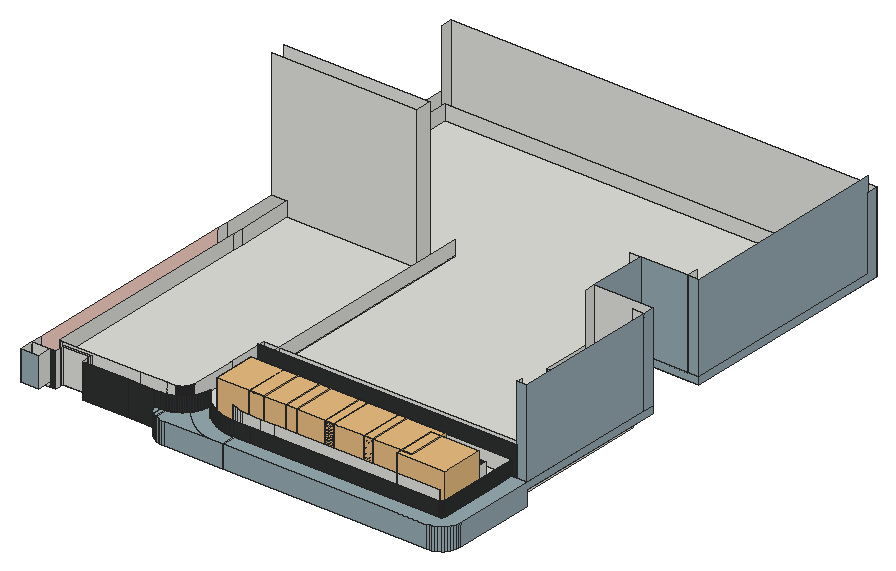
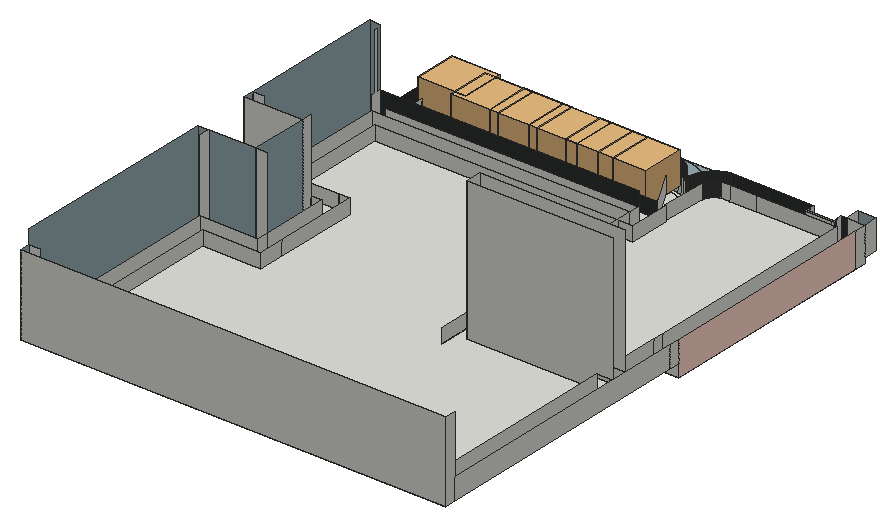
# SketchUp Ruby script. Lengths in inches.
U = 1.inch
M = Sketchup.active_model
def pt(a) = Geom::Point3d.new(a.map { |v| v * U })
def face(e, loops, mat)
  f = e.add_face(loops[0].map { |a| pt(a) })
  loops[1..].each { |l| e.add_face(l.map { |a| pt(a) }).erase! }
  f.material = f.back_material = mat if mat
  f
end
# faces: each face lists its corners as indices into pts; further lists are holes
def faces(e, pts, list, mat = nil) = list.each { |f| face(e, (f[0].is_a?(Array) ? f : [f]).map { |l| l.map { |i| pts[i] } }, mat) }
# xy, xz, yz: faces in a plane at the given z, y or x. An outline is a flat list of corners, or four numbers for a rectangle; further outlines are holes
def ring(l) = l.size == 4 ? [[l[0], l[1]], [l[2], l[1]], [l[2], l[3]], [l[0], l[3]]] : l.each_slice(2).to_a
def flat(e, list, mat, &to3) = list.each { |f| face(e, (f[0].is_a?(Array) ? f : [f]).map { |l| ring(l).map { |u, v| to3.(u, v) } }, mat) }
def xy(e, z, list, mat = nil) = flat(e, list, mat) { |x, y| [x, y, z] }
def xz(e, y, list, mat = nil) = flat(e, list, mat) { |x, z| [x, y, z] }
def yz(e, x, list, mat = nil) = flat(e, list, mat) { |y, z| [x, y, z] }
def lines(e, pts, list) = list.each { |a, b| e.add_line(pt(pts[a]), pt(pts[b])) }
# prism: a flat outline (further loops are holes) pulled along v
def prism(e, loops, v, mat = nil)
  f = face(e, loops, mat); d = Geom::Vector3d.new(v.map { |x| x * U })
  f.pushpull(f.normal.samedirection?(d) ? d.length : -d.length)
end
def box(e, o, s, mat = nil) = prism(e, [[o, [o[0] + s[0], o[1], o[2]], [o[0] + s[0], o[1] + s[1], o[2]], [o[0], o[1] + s[1], o[2]]]], [0, 0, s[2]], mat)
def at(x, y, z, deg = 0) = Geom::Transformation.translation(pt([x, y, z])) * Geom::Transformation.rotation(ORIGIN, Z_AXIS, deg.degrees)
def axes(o, x, y, z) = Geom::Transformation.new([*x, 0, *y, 0, *z, 0, *pt(o).to_a, 1])
def part(name) = M.definitions.add(name)
# library, detail: a bought-in or finely detailed component or shape, given as its bounding box
def library(name, o, s) = part(name).tap { |d| box(d.entities, o, s) }
def detail(e, o, s) = box(e.add_group.entities, o, s)
def put(e, d, t, mat = nil) = e.add_instance(d, t).tap { |i| i.material = mat if mat }
def group(e, t, mat = nil) = e.add_group.tap { |g| g.transformation = t; g.material = mat if mat }.entities
root = M.entities
M.materials.add("Generic").color = [150, 171, 178]
M.materials.add("Generic\#1").color = [47, 50, 50]
M.materials.add("[Color B01]").color = [255, 216, 204]
c1 = library("Tlon Light 650 Ceiling 152 007",[-12.8,-12.8,-3.78],[25.6,25.6,3.58])
c2 = library("Erigeron glaucus 004",[-15.59,-14.45,0.01],[31.39,28.46,21.32])
xy(root,360,[[129.04,30.0625,127.13,30.16,125.24,30.4375,123.38,30.9,121.58,31.54,120.21,32.1875,120.21,35.14,121.14,34.74,122.16,34.4,123.21,34.14,124.25,33.77,125.82,33.38,127.42,33.15,129.11,33.0625,176.86,33.0625,176.86,30.0625],[176.86,30.0625,176.86,33.0625,345.32,33.0625,347.08,33.18,348.73,33.5,349.22,33.67,349.85,33.71,350.48,33.8125,351.09,33.97,351.69,34.19,352.22,34.44,352.22,31.64,351.46,31.27,349.5,30.6,347.48,30.2,345.41,30.0625],[352.22,31.64,352.22,34.44,352.26,34.46,352.81,34.79,353.32,35.17,353.79,35.59,354.22,36.0625,354.6,36.57,354.9375,37.11,355.22,37.68,355.57,38.08,356.5,39.47,357.24,40.97,357.78,42.55,358.1,44.2,358.22,45.96,358.22,114.0625,361.22,114.0625,361.22,45.87,361.08,43.8,360.68,41.78,360.01,39.82,359.1,37.96,357.95,36.25,356.59,34.69,355.03,33.33,353.32,32.18],[120.21,32.1875,119.85,32.36,118.21,33.34,116.67,34.47,116.2,34.9,116.2,38.05,116.61,37.62,117.42,36.9,118.28,36.25,119.19,35.67,120.15,35.16,120.21,35.14],[116.2,34.9,115.25,35.75,113.97,37.17,112.82,38.7,111.84,40.34,111.01,42.0625,113.61,42.0625,114.06,41.08,114.59,40.14,115.19,39.25,115.87,38.4,116.2,38.05]])
xy(root,362,[[179.86,33.0625,179.86,44.93,173.27,45.23,169.71,45.72,166.21,46.54,162.8,47.67,159.51,49.1,156.36,50.83,153.39,52.85,150.61,55.12,148.05,57.64,145.73,60.38,143.67,63.33,136.45,75.96,136.2,64.13,136.13,63.2,136.03,62.26,135.875,61.33,135.68,60.41,135.45,59.5,135.17,58.6,134.85,57.72,134.5,56.85,134.1,56,133.66,55.16,133.1875,54.35,132.68,53.5625,132.13,52.8,131.55,52.06,130.93,51.35,130.28,50.67,129.61,50.01,128.9,49.39,128.16,48.81,127.4,48.26,126.61,47.74,125.81,47.26,124.98,46.82,124.125,46.42,123.26,46.05,122.375,45.73,121.48,45.45,120.57,45.21,119.2,44.91,119.2,45.0625,51.93,45.0625,51.93,51.0625,29.81,51.0625,29.81,45.0625,13.22,45.0625,13.22,231.0625,139.22,231.0625,139.22,126.0625,136.22,126.0625,136.22,111.0625,349.22,111.0625,349.22,33.67,348.73,33.5,347.08,33.18,345.32,33.0625],[176.86,33.0625,176.86,42.0625,173,42.24,169.17,42.77,165.4,43.64,161.73,44.86,158.1875,46.41,154.8,48.27,151.6,50.4375,148.6,52.89,145.85,55.6,143.35,58.55,141.14,61.72,139.22,65.08,139.19,64,139.12,62.92,139,61.85,138.83,60.79,138.61,59.73,138.34,58.6875,138.02,57.66,137.65,56.64,137.24,55.64,136.79,54.67,136.29,53.71,135.74,52.78,135.16,51.87,134.53,51,133.86,50.15,133.15,49.33,132.41,48.55,131.63,47.8,130.82,47.09,129.98,46.42,129.11,45.79,128.2,45.19,127.28,44.64,126.32,44.14,125.35,43.68,124.35,43.26,123.34,42.89,122.3125,42.57,121.27,42.29,120.21,42.0625,120.21,35.14,120.15,35.16,119.19,35.67,118.28,36.25,117.42,36.9,116.61,37.62,116.2,38.05,116.2,42.0625,51.93,42.0625,51.93,45.0625,119.2,45.0625,119.2,44.91,120.57,45.21,121.48,45.45,122.375,45.73,123.26,46.05,124.125,46.42,124.98,46.82,125.81,47.26,126.61,47.74,127.4,48.26,128.16,48.81,128.9,49.39,129.61,50.01,130.28,50.67,130.93,51.35,131.55,52.06,132.13,52.8,132.68,53.5625,133.1875,54.35,133.66,55.16,134.1,56,134.5,56.85,134.85,57.72,135.17,58.6,135.45,59.5,135.68,60.41,135.875,61.33,136.03,62.26,136.13,63.2,136.2,64.13,136.45,75.96,143.67,63.33,145.73,60.38,148.05,57.64,150.61,55.12,153.39,52.85,156.36,50.83,159.51,49.1,162.8,47.67,166.21,46.54,169.71,45.72,173.27,45.23,179.86,44.93,179.86,33.0625],[173.86,33.0625,173.86,39.2,172.72,39.25,168.62,39.82,164.59,40.75,160.66,42.06,156.86,43.71,153.23,45.71,149.8,48.03,146.6,50.65,143.65,53.56,140.97,56.72,140.9,56.82,140.45,55.5625,139.99,54.4375,139.48,53.33,138.91,52.26,138.3,51.2,137.64,50.18,136.93,49.19,136.17,48.24,135.38,47.32,134.54,46.43,133.66,45.59,132.75,44.79,131.8,44.03,130.81,43.32,129.79,42.65,128.75,42.03,127.67,41.46,126.57,40.94,125.45,40.47,124.31,40.05,123.21,39.7,123.21,34.14,122.16,34.4,121.14,34.74,120.21,35.14,120.21,42.0625,121.27,42.29,122.3125,42.57,123.34,42.89,124.35,43.26,125.35,43.68,126.32,44.14,127.28,44.64,128.2,45.19,129.11,45.79,129.98,46.42,130.82,47.09,131.63,47.8,132.41,48.55,133.15,49.33,133.86,50.15,134.53,51,135.16,51.87,135.74,52.78,136.29,53.71,136.79,54.67,137.24,55.64,137.65,56.64,138.02,57.66,138.34,58.6875,138.61,59.73,138.83,60.79,139,61.85,139.12,62.92,139.19,64,139.22,65.08,141.14,61.72,143.35,58.55,145.85,55.6,148.6,52.89,151.6,50.4375,154.8,48.27,158.1875,46.41,161.73,44.86,165.4,43.64,169.17,42.77,173,42.24,176.86,42.0625,176.86,33.0625],[129.11,33.0625,127.42,33.15,125.82,33.38,124.25,33.77,123.21,34.14,123.21,39.7,124.31,40.05,125.45,40.47,126.57,40.94,127.67,41.46,128.75,42.03,129.79,42.65,130.81,43.32,131.8,44.03,132.75,44.79,133.66,45.59,134.54,46.43,135.38,47.32,136.17,48.24,136.93,49.19,137.64,50.18,138.3,51.2,138.91,52.26,139.48,53.33,139.99,54.4375,140.45,55.5625,140.9,56.82,140.97,56.72,143.65,53.56,146.6,50.65,149.8,48.03,153.23,45.71,156.86,43.71,160.66,42.06,164.59,40.75,168.62,39.82,172.72,39.25,173.86,39.2,173.86,33.0625],[349.22,33.67,349.22,111.0625,136.22,111.0625,136.22,126.0625,139.22,126.0625,139.22,114.0625,352.22,114.0625,352.22,34.44,351.69,34.19,351.09,33.97,350.48,33.8125,349.85,33.71],
  [352.22,34.44,352.22,114.0625,358.22,114.0625,358.22,111.0625,355.22,111.0625,355.22,37.68,354.9375,37.11,354.6,36.57,354.22,36.0625,353.79,35.59,353.32,35.17,352.81,34.79,352.26,34.46],[355.22,37.68,355.22,111.0625,358.22,111.0625,358.22,45.96,358.1,44.2,357.78,42.55,357.24,40.97,356.5,39.47,355.57,38.08],[10.22,42.0625,10.22,234.0625,139.22,234.0625,139.22,231.0625,13.22,231.0625,13.22,45.0625,29.81,45.0625,29.81,42.0625],[29.81,49.75,51.93,51.0625],[139.22,123.0625,139.22,126.0625,349.22,126.0625,349.22,231.0625,139.22,231.0625,139.22,234.0625,352.22,234.0625,352.22,123.0625],
  [139.22,126.0625,349.22,231.0625]])
xy(root,366,[[10.22,29.93,25.22,42.0625],[116.2,38.05,115.87,38.4,115.19,39.25,114.59,40.14,114.06,41.08,113.61,42.0625,116.2,42.0625]])
xy(root,372,[[139.22,114.0625,352.22,123.0625],[352.22,114.0625,361.22,123.0625],[352.22,123.0625,361.22,243.0625],[10.22,234.0625,139.22,243.0625],[139.22,234.0625,352.22,243.0625],
  [10.22,243.0625,10.22,465.0625,352.22,465.0625,352.22,300.0625,304.22,300.0625,304.22,243.0625],[304.22,243.0625,313.22,300.0625],[313.22,291.0625,352.22,300.0625],[352.22,291.0625,361.22,474.0625],[10.22,465.0625,352.22,474.0625]])
xy(root,378,[[172.74,30,176.86,30.0625,171.87,30.0625],[189.58,54.22,201.01,54.22,201.01,65.14,175.2,66.32,173.5625,66.54,171.95,66.92,170.38,67.44,168.86,68.1,167.41,68.9,166.04,69.83,164.76,70.875,163.58,72.04,162.51,73.3,161.5625,74.66,152.85,89.91,337.0625,89.91,337.0625,101.34,133.16,101.34,151.89,68.54,153.44,66.32,155.1875,64.26,157.11,62.36,159.2,60.65,161.44,59.14,163.81,57.84,166.29,56.75,168.85,55.9,171.48,55.29,174.16,54.92],[22.94,54.79,118.78,54.79,119.25,54.9375,119.71,55.11,120.16,55.3,120.61,55.51,121.04,55.74,121.47,55.99,121.88,56.26,122.28,56.55,122.66,56.86,123.03,57.18,123.39,57.52,123.73,57.88,124.05,58.25,124.35,58.64,124.64,59.04,124.91,59.45,125.15,59.875,125.38,60.3125,125.59,60.76,125.78,61.21,125.94,61.68,126.09,62.15,126.21,62.625,126.3125,63.11,126.39,63.59,126.45,64.08,126.48,64.57,127.28,101.34,126.49,101.34,126.49,135.79,339.49,135.79,339.49,221.3125,300.49,221.3125,300.49,221.34,291.49,221.34,291.49,312.79,339.49,312.79,339.49,452.34,22.94,452.34,22.94,302.16,130.22,302.16,130.22,289.3,22.94,289.3],[139.22,114.0625,352.22,123.0625],[352.22,114.0625,361.22,234.03],
  [313.22,234.03,361.22,243.0625],[304.22,234.0625,313.22,291.0625],[304.22,291.0625,352.22,300.0625],[352.22,291.0625,361.22,465.0625]])
xy(root,378,[[129.04,30.0625,171.87,30.0625,168.64,30.29,164.57,30.9375,160.58,31.93,156.6875,33.26,152.92,34.93,149.32,36.91,145.89,39.19,142.68,41.76,139.7,44.6,136.98,47.6875,134.53,51,133.86,50.15,133.15,49.33,132.41,48.55,131.63,47.8,130.82,47.09,129.98,46.42,129.11,45.79,128.2,45.19,127.28,44.64,126.32,44.14,125.35,43.68,124.35,43.26,123.34,42.89,122.3125,42.57,121.27,42.29,120.21,42.0625,120.21,32.1875,121.58,31.54,123.38,30.9,125.24,30.4375,127.13,30.16],[171.87,30.0625,176.86,30.0625,176.86,42.0625,173,42.24,169.17,42.77,165.4,43.64,161.73,44.86,158.1875,46.41,154.8,48.27,151.6,50.4375,148.6,52.89,145.85,55.6,143.35,58.55,141.14,61.72,139.22,65.08,139.19,64,139.12,62.92,139,61.85,138.83,60.79,138.61,59.73,138.34,58.6875,138.02,57.66,137.65,56.64,137.24,55.64,136.79,54.67,136.29,53.71,135.74,52.78,135.16,51.87,134.53,51,136.98,47.6875,139.7,44.6,142.68,41.76,145.89,39.19,149.32,36.91,152.92,34.93,156.6875,33.26,160.58,31.93,164.57,30.9375,168.64,30.29],[176.86,30.0625,345.41,30.0625,347.48,30.2,349.5,30.6,351.46,31.27,353.32,32.18,355.03,33.33,356.59,34.69,357.95,36.25,359.1,37.96,360.01,39.82,360.68,41.78,361.08,43.8,361.22,45.87,361.22,114.0625,348.49,114.0625,348.49,45.87,348.47,45.46,348.39,45.07,348.26,44.6875,348.08,44.33,347.86,43.99,347.59,43.6875,347.29,43.42,346.95,43.2,346.59,43.02,346.21,42.89,345.82,42.8125,345.41,42.79,189.58,42.79,176.86,42.0625],[120.21,32.1875,120.21,42.0625,116.2,42.0625,116.2,34.9,116.67,34.47,118.21,33.34,119.85,32.36],[116.2,34.9,116.2,42.0625,111.01,42.0625,111.84,40.34,112.82,38.7,113.97,37.17,115.25,35.75]],"Generic")
xy(root,378,[[201.01,54.22,337.0625,54.22,337.0625,89.91,152.85,89.91,161.5625,74.66,162.51,73.3,163.58,72.04,164.76,70.875,166.04,69.83,167.41,68.9,168.86,68.1,170.38,67.44,171.95,66.92,173.5625,66.54,175.2,66.32,201.01,65.14]],"Generic\#1")
xz(root,29.93,[[10.22,366,25.22,390]],"Generic")
xz(root,30.0625,[[129.04,360,176.86,378],[176.86,360,345.41,378]],"Generic")
xz(root,33.0625,[[129.11,360,173.86,362],[173.86,360,176.86,362],[176.86,360,179.86,362],[179.86,360,345.32,362]])
xz(root,42.0625,[[111.01,360,113.61,362],[10.22,362,25.22,366],[113.61,362,116.2,366],[10.22,366,25.22,390]])
xz(root,42.0625,[[25.22,362,29.81,390],[51.93,362,88.92,390],[88.92,362,111.01,390],[111.01,378,116.2,390],[116.2,378,120.21,390]],"Generic\#1")
xz(root,42.79,[[189.58,378,345.41,390]],"Generic\#1")
xz(root,49.75,[[29.81,362,51.93,390]])
xz(root,51.0625,[[29.81,362,51.93,390]])
xz(root,54.22,[[189.58,378,201.01,390],[201.01,378,337.0625,390]])
xz(root,54.79,[[22.94,378,25.22,390],[25.22,378,88.92,390],[88.92,378,111.01,390],[111.01,378,118.76,390],[118.76,378,118.78,390]])
xz(root,101.34,[[126.49,378,127.28,390]])
xz(root,101.34,[[133.16,378,337.0625,390]],"Generic\#1")
xz(root,114.0625,[[358.22,360,361.22,360,361.22,372,352.22,372,352.22,362,358.22,362],[139.22,362,352.22,372],[139.22,378,348.49,390]])
xz(root,114.0625,[[352.22,378,361.22,450]],"Generic")
xz(root,114.0625,[[348.49,378,352.22,378,352.22,402,139.22,402,139.22,390,348.49,390]],"Generic\#1")
xz(root,123.0625,[[139.22,362,352.22,372],[139.22,378,352.22,390]])
xz(root,135.79,[[126.49,378,339.49,390]])
xz(root,221.3125,[[300.49,378,339.49,390]])
xz(root,221.34,[[291.49,378,300.49,390]])
xz(root,234.03,[[313.22,378,352.22,390],[352.22,378,361.22,450]])
xz(root,234.0625,[[10.22,362,352.22,372],[304.22,378,313.22,390]])
xz(root,243.0625,[[313.22,372,361.22,378],[313.22,378,361.22,450]])
xz(root,289.3,[[22.94,378,130.22,378,130.22,495.3125,10.22,495.3125,10.22,390,22.94,390]])
xz(root,291.0625,[[304.22,378,313.22,450]])
xz(root,291.0625,[[313.22,372,361.22,378],[313.22,378,352.22,450],[352.22,378,361.22,450]],"Generic")
xz(root,300.0625,[[304.22,378,352.22,390]])
xz(root,302.16,[[22.94,378,22.94,390,10.22,390,10.22,495.3125,130.22,495.3125,130.22,378]])
xz(root,312.79,[[291.49,378,339.49,390]])
xz(root,452.34,[[22.94,378,339.49,390]])
xz(root,465.0625,[[352.22,378,361.22,438]])
xz(root,474.0625,[[10.22,372,361.22,438]])
yz(root,10.22,[[42.0625,362,51.0625,390],[29.93,366,42.0625,390],[234.0625,372,243.0625,390],[243.0625,372,465.0625,390],[465.0625,372,474.0625,438]])
yz(root,10.22,[[51.0625,362,234.0625,390]],"[Color B01]")
yz(root,22.94,[[54.79,378,234.0625,390],[234.0625,378,243.0625,390],[243.0625,378,289.3,390],[302.16,378,452.34,390]])
yz(root,25.22,[[29.93,366,42.0625,390]])
yz(root,29.81,[[42.0625,362,46.1,390],[46.1,362,47.72,390],[47.72,362,49.75,390],[49.75,362,51.0625,390]])
yz(root,51.93,[[42.0625,362,46.1,390],[46.1,362,47.72,390],[47.72,362,49.75,390],[49.75,362,51.0625,390]])
yz(root,116.2,[[34.9,360,34.9,378,42.0625,378,42.0625,366,38.05,366,38.05,360],[38.05,362,42.0625,366]])
yz(root,120.21,[[32.1875,360,32.1875,378,42.0625,378,42.0625,362,35.14,362,35.14,360]])
yz(root,126.49,[[101.34,378,135.79,390]])
yz(root,130.22,[[289.3,378,302.16,495.3125]])
yz(root,139.22,[[114.0625,362,123.0625,372],[123.0625,362,317.04,372],[114.0625,372,317.04,378],[114.0625,378,123.0625,390],[123.0625,378,317.04,390]])
yz(root,176.86,[[30.0625,360,30.0625,378,42.0625,378,42.0625,362,33.0625,362,33.0625,360]])
yz(root,291.49,[[221.34,378,291.0625,390],[291.0625,378,312.79,390]])
yz(root,300.49,[[221.3125,378,221.34,390]])
yz(root,304.22,[[234.0625,378,291.0625,390],[291.0625,378,300.0625,390]])
yz(root,313.22,[[234.03,378,234.0625,390],[234.0625,378,243.0625,450]])
yz(root,313.22,[[243.0625,372,291.0625,378],[243.0625,378,291.0625,450]],"Generic")
yz(root,337.0625,[[54.22,378,89.91,390],[89.91,378,101.34,390]])
yz(root,339.49,[[135.79,378,221.3125,390],[312.79,378,452.34,390]])
yz(root,348.49,[[45.87,378,101.34,390],[101.34,378,114.0625,390]],"Generic\#1")
yz(root,352.22,[[123.0625,362,234.0625,372],[114.0625,378,114.0625,402,117.69,402,117.69,448.5625,119.43,448.5625,119.43,402,123.0625,402,123.0625,378],[123.0625,378,234.03,390],[291.0625,378,300.0625,450],[300.0625,378,465.0625,390]])
yz(root,358.22,[[45.96,360,111.0625,362],[111.0625,360,114.0625,362]])
yz(root,361.22,[[45.87,360,114.0625,360,114.0625,372,243.0625,372,243.0625,378,45.87,378],[291.0625,372,474.0625,372,474.0625,438,465.0625,438,465.0625,378,291.0625,378],[114.0625,378,234.03,450],[234.03,378,243.0625,450],[291.0625,378,465.0625,450]],"Generic")
p = [[129.04,30.0625,378],[127.13,30.16,378],[127.13,30.16,360],[129.04,30.0625,360],[347.48,30.2,378],[345.41,30.0625,378],
  [345.41,30.0625,360],[347.48,30.2,360],[125.24,30.4375,378],[125.24,30.4375,360],[349.5,30.6,378],[349.5,30.6,360],
  [123.38,30.9,378],[123.38,30.9,360],[351.46,31.27,378],[351.46,31.27,360],[121.58,31.54,378],[121.58,31.54,360],
  [353.32,32.18,378],[352.22,31.64,360],[353.32,32.18,360],[120.21,32.1875,378],[120.21,32.1875,360],[119.85,32.36,378],
  [119.85,32.36,360],[355.03,33.33,378],[355.03,33.33,360],[118.21,33.34,378],[118.21,33.34,360],[125.82,33.38,362],
  [127.42,33.15,362],[127.42,33.15,360],[125.82,33.38,360],[129.11,33.0625,362],[129.11,33.0625,360],[345.32,33.0625,362],
  [347.08,33.18,362],[347.08,33.18,360],[345.32,33.0625,360],[348.73,33.5,362],[348.73,33.5,360],[116.67,34.47,378],
  [116.67,34.47,360],[356.59,34.69,378],[356.59,34.69,360],[124.25,33.77,362],[124.25,33.77,360],[349.22,33.67,362],
  [349.22,33.67,360],[349.85,33.71,362],[349.85,33.71,360],[350.48,33.8125,362],[350.48,33.8125,360],[123.21,34.14,362],
  [123.21,34.14,360],[351.09,33.97,362],[351.09,33.97,360],[351.69,34.19,362],[351.69,34.19,360],[122.16,34.4,360],
  [122.16,34.4,362],[352.22,34.44,362],[352.22,34.44,360],[121.14,34.74,360],[121.14,34.74,362],[352.26,34.46,362],
  [352.26,34.46,360],[116.2,34.9,378],[116.2,34.9,360],[352.81,34.79,362],[352.81,34.79,360],[120.21,35.14,360],
  [120.21,35.14,362],[357.95,36.25,378],[357.95,36.25,360],[353.32,35.17,362],[353.32,35.17,360],[115.25,35.75,378],
  [115.25,35.75,360],[120.15,35.16,360],[120.15,35.16,362],[119.19,35.67,360],[119.19,35.67,362],[353.79,35.59,362],
  [353.79,35.59,360],[354.22,36.0625,362],[354.22,36.0625,360],[118.28,36.25,360],[118.28,36.25,362],[113.97,37.17,378],
  [113.97,37.17,360],[354.6,36.57,362],[354.6,36.57,360],[117.42,36.9,360],[117.42,36.9,362],[359.1,37.96,378],
  [359.1,37.96,360],[354.9375,37.11,362],[354.9375,37.11,360],[116.61,37.62,360],[116.61,37.62,362],[355.22,37.68,362],
  [355.22,37.68,360],[112.82,38.7,378],[112.82,38.7,360],[116.2,38.05,360],[116.2,38.05,362],[355.57,38.08,362],
  [355.57,38.08,360],[360.01,39.82,378],[360.01,39.82,360],[115.87,38.4,366],[116.2,38.05,366],[115.87,38.4,360],
  [356.5,39.47,362],[356.5,39.47,360],[115.19,39.25,366],[115.19,39.25,360],[111.84,40.34,378],[111.84,40.34,360],
  [114.59,40.14,366],[114.59,40.14,360],[357.24,40.97,362],[357.24,40.97,360],[360.68,41.78,378],[360.68,41.78,360],
  [114.06,41.08,366],[114.06,41.08,360],[111.01,42.0625,378],[111.01,42.0625,362],[111.01,42.0625,360],[357.78,42.55,362],
  [357.78,42.55,360],[113.61,42.0625,366],[113.61,42.0625,360],[113.61,42.0625,362],[361.08,43.8,378],[361.08,43.8,360],
  [358.1,44.2,362],[358.1,44.2,360],[361.22,45.87,378],[361.22,45.87,360],[358.22,45.96,362],[358.22,45.96,360],
  [121.27,42.29,378],[120.21,42.0625,378],[120.21,42.0625,362],[121.27,42.29,362],[176.86,42.0625,378],[173,42.24,378],
  [173,42.24,362],[176.86,42.0625,362],[169.17,42.77,378],[169.17,42.77,362],[122.3125,42.57,378],[122.3125,42.57,362],
  [123.34,42.89,378],[123.34,42.89,362],[165.4,43.64,378],[165.4,43.64,362],[124.35,43.26,378],[124.35,43.26,362],
  [125.35,43.68,378],[125.35,43.68,362],[161.73,44.86,378],[161.73,44.86,362],[126.32,44.14,378],[126.32,44.14,362],
  [127.28,44.64,378],[127.28,44.64,362],[128.2,45.19,378],[128.2,45.19,362],[158.1875,46.41,378],[158.1875,46.41,362],
  [129.11,45.79,378],[129.11,45.79,362],[129.98,46.42,378],[129.98,46.42,362],[130.82,47.09,378],[130.82,47.09,362],
  [154.8,48.27,378],[154.8,48.27,362],[131.63,47.8,378],[131.63,47.8,362],[132.41,48.55,378],[132.41,48.55,362],
  [151.6,50.4375,378],[151.6,50.4375,362],[133.15,49.33,378],[133.15,49.33,362],[133.86,50.15,378],[133.86,50.15,362],
  [134.53,51,378],[134.53,51,362],[148.6,52.89,378],[148.6,52.89,362],[135.16,51.87,378],[135.16,51.87,362],
  [135.74,52.78,378],[135.74,52.78,362],[136.29,53.71,378],[136.29,53.71,362],[145.85,55.6,378],[145.85,55.6,362],
  [136.79,54.67,378],[136.79,54.67,362],[137.24,55.64,378],[137.24,55.64,362],[137.65,56.64,378],[137.65,56.64,362],
  [143.35,58.55,378],[143.35,58.55,362],[138.02,57.66,378],[138.02,57.66,362],[138.34,58.6875,378],[138.34,58.6875,362],
  [141.14,61.72,378],[141.14,61.72,362],[138.61,59.73,378],[138.61,59.73,362],[138.83,60.79,378],[138.83,60.79,362],
  [139,61.85,378],[139,61.85,362],[139.22,65.08,378],[139.22,65.08,362],[139.12,62.92,378],[139.12,62.92,362],
  [139.19,64,378],[139.19,64,362],[121.27,42.29,390],[120.21,42.0625,390],[176.86,42.0625,390],[173,42.24,390],
  [189.58,42.79,378],[189.58,42.79,390],[169.17,42.77,390],[122.3125,42.57,390],[123.34,42.89,390],[165.4,43.64,390],
  [345.41,42.79,378],[345.82,42.8125,378],[345.82,42.8125,390],[345.41,42.79,390],[346.21,42.89,378],[346.21,42.89,390],
  [124.35,43.26,390],[346.59,43.02,378],[346.59,43.02,390],[346.95,43.2,378],[346.95,43.2,390],[347.29,43.42,378],
  [347.29,43.42,390],[125.35,43.68,390],[347.59,43.6875,378],[347.59,43.6875,390],[161.73,44.86,390],[126.32,44.14,390],
  [347.86,43.99,378],[347.86,43.99,390],[348.08,44.33,378],[348.08,44.33,390],[127.28,44.64,390],[348.26,44.6875,378],
  [348.26,44.6875,390],[128.2,45.19,390],[348.39,45.07,378],[348.39,45.07,390],[158.1875,46.41,390],[348.47,45.46,378],
  [348.47,45.46,390],[129.11,45.79,390],[348.49,45.87,378],[348.49,45.87,390],[129.98,46.42,390],[130.82,47.09,390],
  [154.8,48.27,390],[131.63,47.8,390],[132.41,48.55,390],[151.6,50.4375,390],[133.15,49.33,390],[133.86,50.15,390],
  [134.53,51,390],[148.6,52.89,390],[135.16,51.87,390],[135.74,52.78,390],[136.29,53.71,390],[145.85,55.6,390],
  [136.79,54.67,390],[189.58,54.22,378],[174.16,54.92,378],[174.16,54.92,390],[189.58,54.22,390],[137.24,55.64,390],
  [119.25,54.9375,378],[118.78,54.79,378],[118.78,54.79,390],[119.25,54.9375,390],[119.71,55.11,378],[119.71,55.11,390],
  [171.48,55.29,378],[171.48,55.29,390],[120.16,55.3,378],[120.16,55.3,390],[120.61,55.51,378],[120.61,55.51,390],
  [168.85,55.9,378],[168.85,55.9,390],[121.04,55.74,378],[121.04,55.74,390],[137.65,56.64,390],[143.35,58.55,390],
  [121.47,55.99,378],[121.47,55.99,390],[166.29,56.75,378],[166.29,56.75,390],[121.88,56.26,378],[121.88,56.26,390],
  [122.28,56.55,378],[122.28,56.55,390],[122.66,56.86,378],[122.66,56.86,390],[138.02,57.66,390],[163.81,57.84,378],
  [163.81,57.84,390],[123.03,57.18,378],[123.03,57.18,390],[123.39,57.52,378],[123.39,57.52,390],[123.73,57.88,378],
  [123.73,57.88,390],[138.34,58.6875,390],[161.44,59.14,378],[161.44,59.14,390],[124.05,58.25,378],[124.05,58.25,390],
  [124.35,58.64,378],[124.35,58.64,390],[124.64,59.04,378],[124.64,59.04,390],[141.14,61.72,390],[138.61,59.73,390],
  [124.91,59.45,378],[124.91,59.45,390],[159.2,60.65,378],[159.2,60.65,390],[125.15,59.875,378],[125.15,59.875,390],
  [138.83,60.79,390],[125.38,60.3125,378],[125.38,60.3125,390],[125.59,60.76,378],[125.59,60.76,390],[157.11,62.36,378],
  [157.11,62.36,390],[125.78,61.21,378],[125.78,61.21,390],[139,61.85,390],[125.94,61.68,378],[125.94,61.68,390],
  [126.09,62.15,378],[126.09,62.15,390],[139.22,65.08,390],[139.12,62.92,390],[126.21,62.625,378],[126.21,62.625,390],
  [155.1875,64.26,378],[155.1875,64.26,390],[126.3125,63.11,378],[126.3125,63.11,390],[139.19,64,390],[126.39,63.59,378],
  [126.39,63.59,390],[126.45,64.08,378],[126.45,64.08,390],[126.48,64.57,378],[126.48,64.57,390],[153.44,66.32,378],
  [153.44,66.32,390],[127.28,101.34,378],[127.28,101.34,390],[151.89,68.54,378],[151.89,68.54,390],[133.16,101.34,378],
  [133.16,101.34,390]]
faces(root,p,[[0,1,2,3],[4,5,6,7],[1,8,9,2],[10,4,7,11],[8,12,13,9],[14,10,11,15],[12,16,17,13],[18,14,15,19,20],
  [16,21,22,17],[21,23,24,22],[25,18,20,26],[23,27,28,24],[27,41,42,28],[43,25,26,44],[41,67,68,42],[73,43,44,74],
  [67,77,78,68],[77,89,90,78],[95,73,74,96],[89,103,104,90],[109,95,96,110],[103,118,119,104],[124,109,110,125],[118,128,129,130,119],
  [136,124,125,137],[140,136,137,141]],"Generic")
faces(root,p,[[29,30,31,32],[30,33,34,31],[35,36,37,38],[36,39,40,37],[45,29,32,46],[39,47,48,40],[48,47,49,50],[50,49,51,52],
  [53,45,46,54],[52,51,55,56],[56,55,57,58],[59,60,53,54],[58,57,61,62],[63,64,60,59],[61,65,66,62],[65,69,70,66],
  [71,72,64,63],[69,75,76,70],[79,80,72,71],[81,82,80,79],[75,83,84,76],[83,85,86,84],[87,88,82,81],[85,91,92,86],
  [93,94,88,87],[91,97,98,92],[99,100,94,93],[97,101,102,98],[105,106,100,99],[102,101,107,108],[111,112,106,105,113],[108,107,114,115],
  [116,111,113,117],[120,116,117,121],[115,114,122,123],[126,120,121,127],[123,122,131,132],[133,126,127,134,135],[132,131,138,139],[139,138,142,143],
  [144,145,146,147],[148,149,150,151],[149,152,153,150],[154,144,147,155],[156,154,155,157],[152,158,159,153],[160,156,157,161],[162,160,161,163],
  [158,164,165,159],[166,162,163,167],[168,166,167,169],[170,168,169,171],[164,172,173,165],[174,170,171,175],[176,174,175,177],[178,176,177,179],
  [172,180,181,173],[182,178,179,183],[184,182,183,185],[180,186,187,181],[188,184,185,189],[190,188,189,191],[192,190,191,193],[186,194,195,187],
  [196,192,193,197],[198,196,197,199],[200,198,199,201],[194,202,203,195],[204,200,201,205],[206,204,205,207],[208,206,207,209],[202,210,211,203],
  [212,208,209,213],[214,212,213,215],[210,216,217,211],[218,214,215,219],[220,218,219,221],[222,220,221,223],[216,224,225,217],[226,222,223,227],
  [228,226,227,229],[224,228,229,225],[289,290,291,292],[294,295,296,297],[298,294,297,299],[290,300,301,291],[302,298,299,303],[304,302,303,305],
  [300,306,307,301],[308,304,305,309],[312,308,309,313],[306,314,315,307],[316,312,313,317],[318,316,317,319],[320,318,319,321],[314,323,324,315],
  [325,320,321,326],[327,325,326,328],[329,327,328,330],[323,332,333,324],[334,329,330,335],[336,334,335,337],[338,336,337,339],[342,338,339,343],
  [332,344,345,333],[346,342,343,347],[349,346,347,350],[351,349,350,352],[344,353,354,345],[355,351,352,356],[358,355,356,359],[360,358,359,361],
  [364,360,361,365],[353,366,367,354],[368,364,365,369],[371,368,369,372],[373,371,372,374],[375,373,374,376],[366,377,378,367],[379,375,376,380],
  [377,381,382,378],[381,383,384,382]])
faces(root,p,[[145,144,230,231],[149,148,232,233],[148,234,235,232],[152,149,233,236],[144,154,237,230],[154,156,238,237],[158,152,236,239],[240,241,242,243],
  [241,244,245,242],[156,160,246,238],[244,247,248,245],[247,249,250,248],[249,251,252,250],[160,162,253,246],[251,254,255,252],[164,158,239,256],
  [162,166,257,253],[254,258,259,255],[258,260,261,259],[166,168,262,257],[260,263,264,261],[168,170,265,262],[263,266,267,264],[172,164,256,268],
  [266,269,270,267],[170,174,271,265],[269,272,273,270],[174,176,274,271],[176,178,275,274],[180,172,268,276],[178,182,277,275],[182,184,278,277],
  [186,180,276,279],[184,188,280,278],[188,190,281,280],[190,192,282,281],[194,186,279,283],[192,196,284,282],[196,198,285,284],[198,200,286,285],
  [202,194,283,287],[200,204,288,286],[204,206,293,288],[206,208,310,293],[210,202,287,311],[208,212,322,310],[212,214,331,322],[216,210,311,340],
  [214,218,341,331],[218,220,348,341],[220,222,357,348],[224,216,340,362],[222,226,363,357],[226,228,370,363],[228,224,362,370]],"Generic\#1")
put(root,c1,axes([282.43,48.2,362.34],[0.17,0,0],[0,0.17,0],[0,0,0.17]))
put(root,c1,axes([225.55,48.2,362.34],[0.17,0,0],[0,0.17,0],[0,0,0.17]))
put(root,c1,axes([168.68,48.2,362.34],[0.17,0,0],[0,0.17,0],[0,0,0.17]))
put(root,c2,axes([320.76,72.45,377.99],[1.254,0,0],[0,1.254,0],[0,0,1.254]))
put(root,c2,axes([290.13,76.93,377.99],[1.254,0,0],[0,1.254,0],[0,0,1.254]))
put(root,c2,axes([258,76.93,377.99],[1.254,0,0],[0,1.254,0],[0,0,1.254]))
put(root,c2,axes([225.63,76.93,377.99],[1.254,0,0],[0,1.254,0],[0,0,1.254]))
put(root,c2,axes([195.25,76.93,377.99],[1.254,0,0],[0,1.254,0],[0,0,1.254]))
put(root,c2,axes([168.31,77.15,377.99],[1.254,0,0],[0,1.254,0],[0,0,1.254]))
